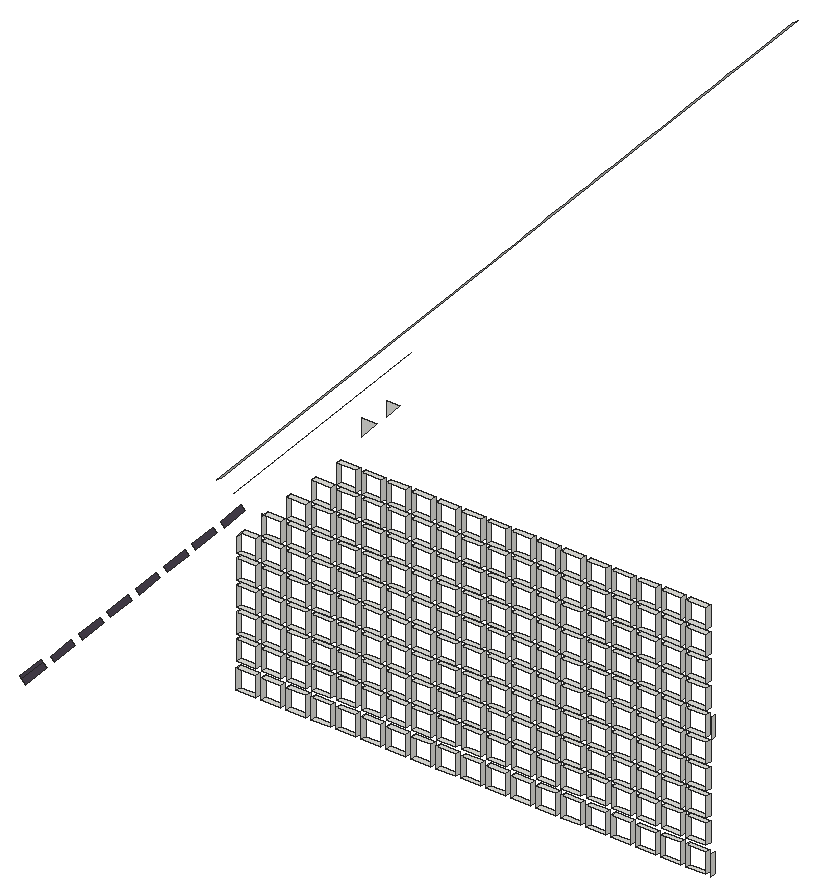
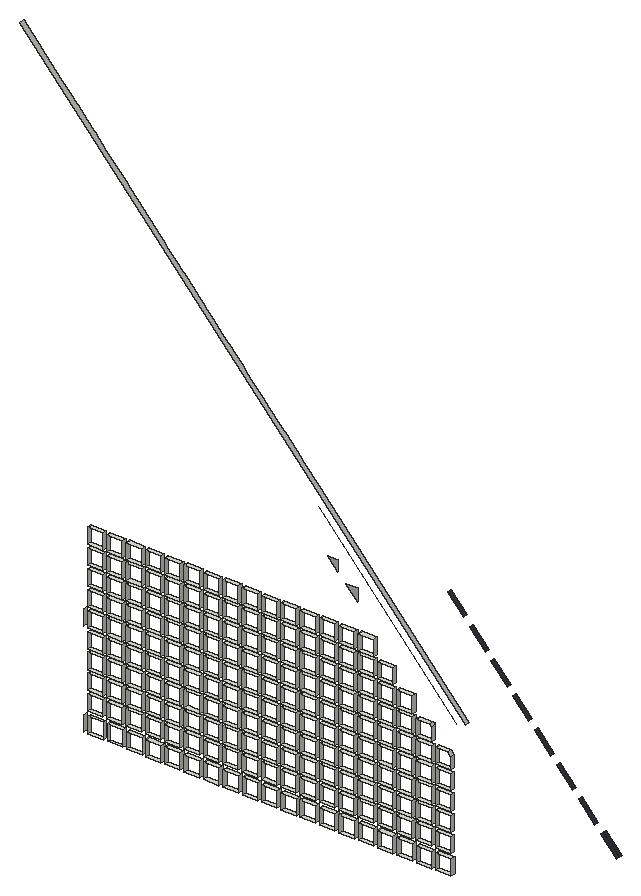
# SketchUp Ruby script. Lengths in inches.
U = 1.inch
M = Sketchup.active_model
def pt(a) = Geom::Point3d.new(a.map { |v| v * U })
def face(e, loops, mat)
  f = e.add_face(loops[0].map { |a| pt(a) })
  loops[1..].each { |l| e.add_face(l.map { |a| pt(a) }).erase! }
  f.material = f.back_material = mat if mat
  f
end
# faces: each face lists its corners as indices into pts; further lists are holes
def faces(e, pts, list, mat = nil) = list.each { |f| face(e, (f[0].is_a?(Array) ? f : [f]).map { |l| l.map { |i| pts[i] } }, mat) }
# xy, xz, yz: faces in a plane at the given z, y or x. An outline is a flat list of corners, or four numbers for a rectangle; further outlines are holes
def ring(l) = l.size == 4 ? [[l[0], l[1]], [l[2], l[1]], [l[2], l[3]], [l[0], l[3]]] : l.each_slice(2).to_a
def flat(e, list, mat, &to3) = list.each { |f| face(e, (f[0].is_a?(Array) ? f : [f]).map { |l| ring(l).map { |u, v| to3.(u, v) } }, mat) }
def xy(e, z, list, mat = nil) = flat(e, list, mat) { |x, y| [x, y, z] }
def xz(e, y, list, mat = nil) = flat(e, list, mat) { |x, z| [x, y, z] }
def yz(e, x, list, mat = nil) = flat(e, list, mat) { |y, z| [x, y, z] }
def lines(e, pts, list) = list.each { |a, b| e.add_line(pt(pts[a]), pt(pts[b])) }
# prism: a flat outline (further loops are holes) pulled along v
def prism(e, loops, v, mat = nil)
  f = face(e, loops, mat); d = Geom::Vector3d.new(v.map { |x| x * U })
  f.pushpull(f.normal.samedirection?(d) ? d.length : -d.length)
end
def box(e, o, s, mat = nil) = prism(e, [[o, [o[0] + s[0], o[1], o[2]], [o[0] + s[0], o[1] + s[1], o[2]], [o[0], o[1] + s[1], o[2]]]], [0, 0, s[2]], mat)
def at(x, y, z, deg = 0) = Geom::Transformation.translation(pt([x, y, z])) * Geom::Transformation.rotation(ORIGIN, Z_AXIS, deg.degrees)
def axes(o, x, y, z) = Geom::Transformation.new([*x, 0, *y, 0, *z, 0, *pt(o).to_a, 1])
def part(name) = M.definitions.add(name)
# library, detail: a bought-in or finely detailed component or shape, given as its bounding box
def library(name, o, s) = part(name).tap { |d| box(d.entities, o, s) }
def detail(e, o, s) = box(e.add_group.entities, o, s)
def put(e, d, t, mat = nil) = e.add_instance(d, t).tap { |i| i.material = mat if mat }
def group(e, t, mat = nil) = e.add_group.tap { |g| g.transformation = t; g.material = mat if mat }.entities
root = M.entities
M.materials.add("[Color M06]").color = [79, 71, 84]
xy(root,305.35,[[433.17,480.14,435.48,480.77],[436.08,480.14,438.39,480.77],[438.99,480.14,441.31,480.77],[441.91,480.14,444.22,480.77],[444.82,480.14,447.13,480.77],
  [447.73,480.14,450.04,480.77],[450.64,480.14,452.95,480.77],[453.55,480.14,455.87,480.77],[456.47,480.14,458.78,480.77],[459.38,480.14,461.69,480.77],
  [462.29,480.14,464.6,480.77],[465.2,480.14,467.51,480.77],[468.11,480.14,470.43,480.77],[471.03,480.14,473.34,480.77],[473.9375,480.14,476.25,480.77],
  [476.85,480.14,479.16,480.77],[479.76,480.14,482.07,480.64],[482.67,480.14,484.99,480.64],[485.59,480.14,487.9,480.64]])
xy(root,307.67,[[433.17,480.14,435.48,480.77],[436.08,480.14,438.39,480.77],[438.99,480.14,441.31,480.77],[441.91,480.14,444.22,480.77],[444.82,480.14,447.13,480.77],
  [447.73,480.14,450.04,480.77],[450.64,480.14,452.95,480.77],[453.55,480.14,455.87,480.77],[456.47,480.14,458.78,480.77],[459.38,480.14,461.69,480.77],
  [462.29,480.14,464.6,480.77],[465.2,480.14,467.51,480.77],[468.11,480.14,470.43,480.77],[471.03,480.14,473.34,480.77],[473.9375,480.14,476.25,480.77],
  [476.85,480.14,479.16,480.77],[479.76,480.14,482.07,480.64],[482.67,480.14,484.99,480.64],[485.59,480.14,487.9,480.64]])
xy(root,308.4,[[433.2,480.14,435.51,480.77],[436.11,480.14,438.42,480.77],[439.02,480.14,441.33,480.77],[441.93,480.14,444.25,480.77],[444.85,480.14,447.16,480.77],
  [447.76,480.14,450.07,480.77],[450.67,480.14,452.98,480.77],[453.58,480.14,455.89,480.77],[456.49,480.14,458.81,480.77],[459.41,480.14,461.72,480.77],
  [462.32,480.14,464.63,480.77],[465.23,480.14,467.54,480.77],[468.14,480.14,470.45,480.77],[471.05,480.14,473.37,480.77],[473.97,480.14,476.28,480.77],
  [476.88,480.14,479.19,480.77],[479.79,480.14,482.1,480.77],[482.7,480.14,485.02,480.77],[485.61,480.14,487.93,480.77]])
xy(root,310.71,[[433.2,480.14,435.51,480.77],[436.11,480.14,438.42,480.77],[439.02,480.14,441.33,480.77],[441.93,480.14,444.25,480.77],[444.85,480.14,447.16,480.77],
  [447.76,480.14,450.07,480.77],[450.67,480.14,452.98,480.77],[453.58,480.14,455.89,480.77],[456.49,480.14,458.81,480.77],[459.41,480.14,461.72,480.77],
  [462.32,480.14,464.63,480.77],[465.23,480.14,467.54,480.77],[468.14,480.14,470.45,480.77],[471.05,480.14,473.37,480.77],[473.97,480.14,476.28,480.77],
  [476.88,480.14,479.19,480.77],[479.79,480.14,482.1,480.77],[482.7,480.14,485.02,480.77],[485.61,480.14,487.93,480.77]])
xy(root,311.21,[[433.2,480.14,435.51,480.77],[436.11,480.14,438.42,480.77],[439.02,480.14,441.33,480.77],[441.93,480.14,444.25,480.77],[444.85,480.14,447.16,480.77],
  [447.76,480.14,450.07,480.77],[450.67,480.14,452.98,480.77],[453.58,480.14,455.89,480.77],[456.49,480.14,458.81,480.77],[459.41,480.14,461.72,480.77],
  [462.32,480.14,464.63,480.77],[465.23,480.14,467.54,480.77],[468.14,480.14,470.45,480.77],[471.05,480.14,473.37,480.77],[473.97,480.14,476.28,480.77],
  [476.88,480.14,479.19,480.77],[479.79,480.14,482.1,480.77],[482.7,480.14,485.02,480.77],[485.61,480.14,487.93,480.77]])
xy(root,313.52,[[433.2,480.14,435.51,480.77],[436.11,480.14,438.42,480.77],[439.02,480.14,441.33,480.77],[441.93,480.14,444.25,480.77],[444.85,480.14,447.16,480.77],
  [447.76,480.14,450.07,480.77],[450.67,480.14,452.98,480.77],[453.58,480.14,455.89,480.77],[456.49,480.14,458.81,480.77],[459.41,480.14,461.72,480.77],
  [462.32,480.14,464.63,480.77],[465.23,480.14,467.54,480.77],[468.14,480.14,470.45,480.77],[471.05,480.14,473.37,480.77],[473.97,480.14,476.28,480.77],
  [476.88,480.14,479.19,480.77],[479.79,480.14,482.1,480.77],[482.7,480.14,485.02,480.77],[485.61,480.14,487.93,480.77]])
xy(root,314.02,[[433.2,480.14,435.51,480.77],[436.11,480.14,438.42,480.77],[439.02,480.14,441.33,480.77],[441.93,480.14,444.25,480.77],[444.85,480.14,447.16,480.77],
  [447.76,480.14,450.07,480.77],[450.67,480.14,452.98,480.77],[453.58,480.14,455.89,480.77],[456.49,480.14,458.81,480.77],[459.41,480.14,461.72,480.77],
  [462.32,480.14,464.63,480.77],[465.23,480.14,467.54,480.77],[468.14,480.14,470.45,480.77],[471.05,480.14,473.37,480.77],[473.97,480.14,476.28,480.77],
  [476.88,480.14,479.19,480.77],[479.79,480.14,482.1,480.77],[482.7,480.14,485.02,480.77],[485.61,480.14,487.93,480.77]])
xy(root,316.34,[[433.2,480.14,435.51,480.77],[436.11,480.14,438.42,480.77],[439.02,480.14,441.33,480.77],[441.93,480.14,444.25,480.77],[444.85,480.14,447.16,480.77],
  [447.76,480.14,450.07,480.77],[450.67,480.14,452.98,480.77],[453.58,480.14,455.89,480.77],[456.49,480.14,458.81,480.77],[459.41,480.14,461.72,480.77],
  [462.32,480.14,464.63,480.77],[465.23,480.14,467.54,480.77],[468.14,480.14,470.45,480.77],[471.05,480.14,473.37,480.77],[473.97,480.14,476.28,480.77],
  [476.88,480.14,479.19,480.77],[479.79,480.14,482.1,480.77],[482.7,480.14,485.02,480.77],[485.61,480.14,487.93,480.77]])
xy(root,316.84,[[433.2,480.14,435.51,480.77],[436.11,480.14,438.42,480.77],[439.02,480.14,441.33,480.77],[441.93,480.14,444.25,480.77],[444.85,480.14,447.16,480.77],
  [447.76,480.14,450.07,480.77],[450.67,480.14,452.98,480.77],[453.58,480.14,455.89,480.77],[456.49,480.14,458.81,480.77],[459.41,480.14,461.72,480.77],
  [462.32,480.14,464.63,480.77],[465.23,480.14,467.54,480.77],[468.14,480.14,470.45,480.77],[471.05,480.14,473.37,480.77],[473.97,480.14,476.28,480.77],
  [476.88,480.14,479.19,480.77],[479.79,480.14,482.1,480.77],[482.7,480.14,485.02,480.77],[485.61,480.14,487.93,480.77]])
xy(root,319.15,[[433.2,480.14,435.51,480.77],[436.11,480.14,438.42,480.77],[439.02,480.14,441.33,480.77],[441.93,480.14,444.25,480.77],[444.85,480.14,447.16,480.77],
  [447.76,480.14,450.07,480.77],[450.67,480.14,452.98,480.77],[453.58,480.14,455.89,480.77],[456.49,480.14,458.81,480.77],[459.41,480.14,461.72,480.77],
  [462.32,480.14,464.63,480.77],[465.23,480.14,467.54,480.77],[468.14,480.14,470.45,480.77],[471.05,480.14,473.37,480.77],[473.97,480.14,476.28,480.77],
  [476.88,480.14,479.19,480.77],[479.79,480.14,482.1,480.77],[482.7,480.14,485.02,480.77],[485.61,480.14,487.93,480.77]])
xy(root,319.65,[[433.2,480.14,435.51,480.77],[436.11,480.14,438.42,480.77],[439.02,480.14,441.33,480.77],[441.93,480.14,444.25,480.77],[444.85,480.14,447.16,480.77],
  [447.76,480.14,450.07,480.77],[450.67,480.14,452.98,480.77],[453.58,480.14,455.89,480.77],[456.49,480.14,458.81,480.77],[459.41,480.14,461.72,480.77],
  [462.32,480.14,464.63,480.77],[465.23,480.14,467.54,480.77],[468.14,480.14,470.45,480.77],[471.05,480.14,473.37,480.77],[473.97,480.14,476.28,480.77],
  [476.88,480.14,479.19,480.77],[479.79,480.14,482.1,480.77],[482.7,480.14,485.02,480.77],[485.61,480.14,487.93,480.7]])
xy(root,321.96,[[433.73,480.14,435.51,480.77],[436.11,480.14,438.42,480.77],[439.02,480.14,441.33,480.77],[441.93,480.14,444.25,480.77],[444.85,480.14,447.16,480.77],
  [447.76,480.14,450.07,480.77],[450.67,480.14,452.98,480.77],[453.58,480.14,455.89,480.77],[456.49,480.14,458.81,480.77],[459.41,480.14,461.72,480.77],
  [462.32,480.14,464.63,480.77],[465.23,480.14,467.54,480.77],[468.14,480.14,470.45,480.77],[471.05,480.14,473.37,480.77],[473.97,480.14,476.28,480.77],
  [476.88,480.14,479.19,480.77],[479.79,480.14,482.1,480.77],[482.7,480.14,485.02,480.77],[485.61,480.14,487.93,480.7]])
xy(root,322.46,[[436.11,480.14,438.42,480.77],[439.02,480.14,441.33,480.77],[441.93,480.14,444.25,480.77],[444.85,480.14,447.16,480.77],[447.76,480.14,450.07,480.77],
  [450.67,480.14,452.98,480.77],[453.58,480.14,455.89,480.77],[456.49,480.14,458.81,480.77],[459.41,480.14,461.72,480.77],[462.32,480.14,464.63,480.77],
  [465.23,480.14,467.54,480.77],[468.14,480.14,470.45,480.77],[471.05,480.14,473.37,480.77],[473.97,480.14,476.28,480.77],[476.88,480.14,479.19,480.77],
  [479.79,480.14,482.1,480.77],[482.7,480.14,485.02,480.77],[485.61,480.14,487.93,480.77]])
xy(root,324.77,[[436.37,480.14,438.42,480.77],[439.02,480.14,441.33,480.77],[441.93,480.14,444.25,480.77],[444.85,480.14,447.16,480.77],[447.76,480.14,450.07,480.77],
  [450.67,480.14,452.98,480.77],[453.58,480.14,455.89,480.77],[456.49,480.14,458.81,480.77],[459.41,480.14,461.72,480.77],[462.32,480.14,464.63,480.77],
  [465.23,480.14,467.54,480.77],[468.14,480.14,470.45,480.77],[471.05,480.14,473.37,480.77],[473.97,480.14,476.28,480.77],[476.88,480.14,479.19,480.77],
  [479.79,480.14,482.1,480.77],[482.7,480.14,485.02,480.77],[485.61,480.14,487.93,480.77]])
xy(root,325.27,[[439.02,480.14,441.33,480.77],[441.93,480.14,444.25,480.77],[444.85,480.14,447.16,480.77],[447.76,480.14,450.07,480.77],[450.67,480.14,452.98,480.77],
  [453.58,480.14,455.89,480.77],[456.49,480.14,458.81,480.77],[459.41,480.14,461.72,480.77],[462.32,480.14,464.63,480.77],[465.23,480.14,467.54,480.77],
  [468.14,480.14,470.45,480.77],[471.05,480.14,473.37,480.77],[473.97,480.14,476.28,480.77],[476.88,480.14,479.19,480.77],[479.79,480.14,482.1,480.77],
  [482.7,480.14,485.02,480.77],[485.61,480.14,487.93,480.77]])
xy(root,327.59,[[439.02,480.14,441.33,480.77],[441.93,480.14,444.25,480.77],[444.85,480.14,447.16,480.77],[447.76,480.14,450.07,480.77],[450.67,480.14,452.98,480.77],
  [453.58,480.14,455.89,480.77],[456.49,480.14,458.81,480.77],[459.41,480.14,461.72,480.77],[462.32,480.14,464.63,480.77],[465.23,480.14,467.54,480.77],
  [468.14,480.14,470.45,480.77],[471.05,480.14,473.37,480.77],[473.97,480.14,476.28,480.77],[476.88,480.14,479.19,480.77],[479.79,480.14,482.1,480.77],
  [482.7,480.14,485.02,480.77],[485.61,480.14,487.93,480.77]])
xy(root,328.09,[[441.93,480.14,444.25,480.77],[444.85,480.14,447.16,480.77],[447.76,480.14,450.07,480.77],[450.67,480.14,452.98,480.77],[453.58,480.14,455.89,480.77],
  [456.49,480.14,458.81,480.77],[459.41,480.14,461.72,480.77],[462.32,480.14,464.63,480.77],[465.23,480.14,467.54,480.77],[468.14,480.14,470.45,480.77],
  [471.05,480.14,473.37,480.77],[473.97,480.14,476.28,480.77],[476.88,480.14,479.19,480.77],[479.79,480.14,482.1,480.77],[482.7,480.14,485.02,480.77],
  [485.61,480.14,487.93,480.77]])
xy(root,330.4,[[441.93,480.14,444.25,480.77],[444.85,480.14,447.16,480.77],[447.76,480.14,450.07,480.77],[450.67,480.14,452.98,480.77],[453.58,480.14,455.89,480.77],
  [456.49,480.14,458.81,480.77],[459.41,480.14,461.72,480.77],[462.32,480.14,464.63,480.77],[465.23,480.14,467.54,480.77],[468.14,480.14,470.45,480.77],
  [471.05,480.14,473.37,480.77],[473.97,480.14,476.28,480.77],[476.88,480.14,479.19,480.77],[479.79,480.14,482.1,480.77],[482.7,480.14,485.02,480.77],
  [485.61,480.14,487.93,480.77]])
xy(root,330.9,[[444.85,480.14,447.16,480.77],[447.76,480.14,450.07,480.77],[450.67,480.14,452.98,480.77],[453.58,480.14,455.89,480.77],[456.49,480.14,458.81,480.77],
  [459.41,480.14,461.72,480.77],[462.32,480.14,464.63,480.77],[465.23,480.14,467.54,480.77],[468.14,480.14,470.45,480.77],[471.05,480.14,473.37,480.77],
  [473.97,480.14,476.28,480.77],[476.88,480.14,479.19,480.77],[479.79,480.14,482.1,480.77],[482.7,480.14,485.02,480.77],[485.61,480.14,487.93,480.77]])
xy(root,333.21,[[444.85,480.14,447.16,480.77],[447.76,480.14,450.07,480.77],[450.67,480.14,452.98,480.77],[453.58,480.14,455.89,480.77],[456.49,480.14,458.81,480.77],
  [459.41,480.14,461.72,480.77],[462.32,480.14,464.63,480.77],[465.23,480.14,467.54,480.77],[468.14,480.14,470.45,480.77],[471.05,480.14,473.37,480.77],
  [473.97,480.14,476.28,480.77],[476.88,480.14,479.19,480.77],[479.79,480.14,482.1,480.77],[482.7,480.14,485.02,480.77],[485.61,480.14,487.93,480.77]])
xz(root,467.1875,[[419.07,306.65,421.49,309.22,421.04,309.65,418.61,307.08],[418.61,307.08,421.04,309.65,420.81,309.87,418.39,307.29],[422.37,310.16,424.79,312.73,424.33,313.16,421.91,310.59],[425.67,313.66,428.09,316.23,427.63,316.66,425.21,314.09],[428.96,317.17,431.39,319.74,430.93,320.17,428.51,317.59],
  [432.26,320.67,434.68,323.24,434.23,323.67,431.81,321.1],[435.5625,324.17,437.98,326.75,437.53,327.17,435.11,324.6],[438.86,327.68,441.28,330.25,440.83,330.68,438.41,328.11],[442.16,331.18,444.58,333.75,444.125,334.18,441.7,331.61]],"[Color M06]")
xz(root,480.14,[[436.11,324.5,436.37,324.77,436.11,324.77],[447.76,336.93,449.55,338.84,447.76,338.84],[450.67,340.04,452.18,341.65,450.67,341.65]])
yz(root,433.17,[[480.14,305.35,480.77,307.67]])
yz(root,433.2,[[480.14,308.4,480.77,310.71],[480.14,311.21,480.77,313.52],[480.14,314.02,480.77,316.34],[480.14,316.84,480.77,319.15],[480.14,319.65,480.77,321.39]])
yz(root,435.48,[[480.14,305.35,480.77,307.67]])
yz(root,435.51,[[480.14,308.4,480.77,310.71],[480.14,311.21,480.77,313.52],[480.14,314.02,480.77,316.34],[480.14,316.84,480.77,319.15],[480.14,319.65,480.77,321.96]])
yz(root,436.08,[[480.14,305.35,480.77,307.67]])
yz(root,436.11,[[480.14,308.4,480.77,310.71],[480.14,311.21,480.77,313.52],[480.14,314.02,480.77,316.34],[480.14,316.84,480.77,319.15],[480.14,319.65,480.77,321.96],
  [480.14,322.46,480.77,324.5]])
yz(root,438.39,[[480.14,305.35,480.77,307.67]])
yz(root,438.42,[[480.14,308.4,480.77,310.71],[480.14,311.21,480.77,313.52],[480.14,314.02,480.77,316.34],[480.14,316.84,480.77,319.15],[480.14,319.65,480.77,321.96],
  [480.14,322.46,480.77,324.77]])
yz(root,438.99,[[480.14,305.35,480.77,307.67]])
yz(root,439.02,[[480.14,308.4,480.77,310.71],[480.14,311.21,480.77,313.52],[480.14,314.02,480.77,316.34],[480.14,316.84,480.77,319.15],[480.14,319.65,480.77,321.96],
  [480.14,322.46,480.77,324.77],[480.14,325.27,480.77,327.59]])
yz(root,441.31,[[480.14,305.35,480.77,307.67]])
yz(root,441.33,[[480.14,308.4,480.77,310.71],[480.14,311.21,480.77,313.52],[480.14,314.02,480.77,316.34],[480.14,316.84,480.77,319.15],[480.14,319.65,480.77,321.96],
  [480.14,322.46,480.77,324.77],[480.14,325.27,480.77,327.59]])
yz(root,441.91,[[480.14,305.35,480.77,307.67]])
yz(root,441.93,[[480.14,308.4,480.77,310.71],[480.14,311.21,480.77,313.52],[480.14,314.02,480.77,316.34],[480.14,316.84,480.77,319.15],[480.14,319.65,480.77,321.96],
  [480.14,322.46,480.77,324.77],[480.14,325.27,480.77,327.59],[480.14,328.09,480.77,330.4]])
yz(root,444.22,[[480.14,305.35,480.77,307.67]])
yz(root,444.25,[[480.14,308.4,480.77,310.71],[480.14,311.21,480.77,313.52],[480.14,314.02,480.77,316.34],[480.14,316.84,480.77,319.15],[480.14,319.65,480.77,321.96],
  [480.14,322.46,480.77,324.77],[480.14,325.27,480.77,327.59],[480.14,328.09,480.77,330.4]])
yz(root,444.82,[[480.14,305.35,480.77,307.67]])
yz(root,444.85,[[480.14,308.4,480.77,310.71],[480.14,311.21,480.77,313.52],[480.14,314.02,480.77,316.34],[480.14,316.84,480.77,319.15],[480.14,319.65,480.77,321.96],
  [480.14,322.46,480.77,324.77],[480.14,325.27,480.77,327.59],[480.14,328.09,480.77,330.4],[480.14,330.9,480.77,333.21]])
yz(root,447.13,[[480.14,305.35,480.77,307.67]])
yz(root,447.16,[[480.14,308.4,480.77,310.71],[480.14,311.21,480.77,313.52],[480.14,314.02,480.77,316.34],[480.14,316.84,480.77,319.15],[480.14,319.65,480.77,321.96],
  [480.14,322.46,480.77,324.77],[480.14,325.27,480.77,327.59],[480.14,328.09,480.77,330.4],[480.14,330.9,480.77,333.21]])
yz(root,447.73,[[480.14,305.35,480.77,307.67]])
yz(root,447.76,[[480.14,308.4,480.77,310.71],[480.14,311.21,480.77,313.52],[480.14,314.02,480.77,316.34],[480.14,316.84,480.77,319.15],[480.14,319.65,480.77,321.96],
  [480.14,322.46,480.77,324.77],[480.14,325.27,480.77,327.59],[480.14,328.09,480.77,330.4],[480.14,330.9,480.77,333.21]])
yz(root,450.04,[[480.14,305.35,480.77,307.67]])
yz(root,450.07,[[480.14,308.4,480.77,310.71],[480.14,311.21,480.77,313.52],[480.14,314.02,480.77,316.34],[480.14,316.84,480.77,319.15],[480.14,319.65,480.77,321.96],
  [480.14,322.46,480.77,324.77],[480.14,325.27,480.77,327.59],[480.14,328.09,480.77,330.4],[480.14,330.9,480.77,333.21]])
yz(root,450.64,[[480.14,305.35,480.77,307.67]])
yz(root,450.67,[[480.14,308.4,480.77,310.71],[480.14,311.21,480.77,313.52],[480.14,314.02,480.77,316.34],[480.14,316.84,480.77,319.15],[480.14,319.65,480.77,321.96],
  [480.14,322.46,480.77,324.77],[480.14,325.27,480.77,327.59],[480.14,328.09,480.77,330.4],[480.14,330.9,480.77,333.21]])
yz(root,452.95,[[480.14,305.35,480.77,307.67]])
yz(root,452.98,[[480.14,308.4,480.77,310.71],[480.14,311.21,480.77,313.52],[480.14,314.02,480.77,316.34],[480.14,316.84,480.77,319.15],[480.14,319.65,480.77,321.96],
  [480.14,322.46,480.77,324.77],[480.14,325.27,480.77,327.59],[480.14,328.09,480.77,330.4],[480.14,330.9,480.77,333.21]])
yz(root,453.55,[[480.14,305.35,480.77,307.67]])
yz(root,453.58,[[480.14,308.4,480.77,310.71],[480.14,311.21,480.77,313.52],[480.14,314.02,480.77,316.34],[480.14,316.84,480.77,319.15],[480.14,319.65,480.77,321.96],
  [480.14,322.46,480.77,324.77],[480.14,325.27,480.77,327.59],[480.14,328.09,480.77,330.4],[480.14,330.9,480.77,333.21]])
yz(root,455.87,[[480.14,305.35,480.77,307.67]])
yz(root,455.89,[[480.14,308.4,480.77,310.71],[480.14,311.21,480.77,313.52],[480.14,314.02,480.77,316.34],[480.14,316.84,480.77,319.15],[480.14,319.65,480.77,321.96],
  [480.14,322.46,480.77,324.77],[480.14,325.27,480.77,327.59],[480.14,328.09,480.77,330.4],[480.14,330.9,480.77,333.21]])
yz(root,456.47,[[480.14,305.35,480.77,307.67]])
yz(root,456.49,[[480.14,308.4,480.77,310.71],[480.14,311.21,480.77,313.52],[480.14,314.02,480.77,316.34],[480.14,316.84,480.77,319.15],[480.14,319.65,480.77,321.96],
  [480.14,322.46,480.77,324.77],[480.14,325.27,480.77,327.59],[480.14,328.09,480.77,330.4],[480.14,330.9,480.77,333.21]])
yz(root,458.78,[[480.14,305.35,480.77,307.67]])
yz(root,458.81,[[480.14,308.4,480.77,310.71],[480.14,311.21,480.77,313.52],[480.14,314.02,480.77,316.34],[480.14,316.84,480.77,319.15],[480.14,319.65,480.77,321.96],
  [480.14,322.46,480.77,324.77],[480.14,325.27,480.77,327.59],[480.14,328.09,480.77,330.4],[480.14,330.9,480.77,333.21]])
yz(root,459.38,[[480.14,305.35,480.77,307.67]])
yz(root,459.41,[[480.14,308.4,480.77,310.71],[480.14,311.21,480.77,313.52],[480.14,314.02,480.77,316.34],[480.14,316.84,480.77,319.15],[480.14,319.65,480.77,321.96],
  [480.14,322.46,480.77,324.77],[480.14,325.27,480.77,327.59],[480.14,328.09,480.77,330.4],[480.14,330.9,480.77,333.21]])
yz(root,461.69,[[480.14,305.35,480.77,307.67]])
yz(root,461.72,[[480.14,308.4,480.77,310.71],[480.14,311.21,480.77,313.52],[480.14,314.02,480.77,316.34],[480.14,316.84,480.77,319.15],[480.14,319.65,480.77,321.96],
  [480.14,322.46,480.77,324.77],[480.14,325.27,480.77,327.59],[480.14,328.09,480.77,330.4],[480.14,330.9,480.77,333.21]])
yz(root,462.29,[[480.14,305.35,480.77,307.67]])
yz(root,462.32,[[480.14,308.4,480.77,310.71],[480.14,311.21,480.77,313.52],[480.14,314.02,480.77,316.34],[480.14,316.84,480.77,319.15],[480.14,319.65,480.77,321.96],
  [480.14,322.46,480.77,324.77],[480.14,325.27,480.77,327.59],[480.14,328.09,480.77,330.4],[480.14,330.9,480.77,333.21]])
yz(root,464.6,[[480.14,305.35,480.77,307.67]])
yz(root,464.63,[[480.14,308.4,480.77,310.71],[480.14,311.21,480.77,313.52],[480.14,314.02,480.77,316.34],[480.14,316.84,480.77,319.15],[480.14,319.65,480.77,321.96],
  [480.14,322.46,480.77,324.77],[480.14,325.27,480.77,327.59],[480.14,328.09,480.77,330.4],[480.14,330.9,480.77,333.21]])
yz(root,465.2,[[480.14,305.35,480.77,307.67]])
yz(root,465.23,[[480.14,308.4,480.77,310.71],[480.14,311.21,480.77,313.52],[480.14,314.02,480.77,316.34],[480.14,316.84,480.77,319.15],[480.14,319.65,480.77,321.96],
  [480.14,322.46,480.77,324.77],[480.14,325.27,480.77,327.59],[480.14,328.09,480.77,330.4],[480.14,330.9,480.77,333.21]])
yz(root,467.51,[[480.14,305.35,480.77,307.67]])
yz(root,467.54,[[480.14,308.4,480.77,310.71],[480.14,311.21,480.77,313.52],[480.14,314.02,480.77,316.34],[480.14,316.84,480.77,319.15],[480.14,319.65,480.77,321.96],
  [480.14,322.46,480.77,324.77],[480.14,325.27,480.77,327.59],[480.14,328.09,480.77,330.4],[480.14,330.9,480.77,333.21]])
yz(root,468.11,[[480.14,305.35,480.77,307.67]])
yz(root,468.14,[[480.14,308.4,480.77,310.71],[480.14,311.21,480.77,313.52],[480.14,314.02,480.77,316.34],[480.14,316.84,480.77,319.15],[480.14,319.65,480.77,321.96],
  [480.14,322.46,480.77,324.77],[480.14,325.27,480.77,327.59],[480.14,328.09,480.77,330.4],[480.14,330.9,480.77,333.21]])
yz(root,470.43,[[480.14,305.35,480.77,307.67]])
yz(root,470.45,[[480.14,308.4,480.77,310.71],[480.14,311.21,480.77,313.52],[480.14,314.02,480.77,316.34],[480.14,316.84,480.77,319.15],[480.14,319.65,480.77,321.96],
  [480.14,322.46,480.77,324.77],[480.14,325.27,480.77,327.59],[480.14,328.09,480.77,330.4],[480.14,330.9,480.77,333.21]])
yz(root,471.03,[[480.14,305.35,480.77,307.67]])
yz(root,471.05,[[480.14,308.4,480.77,310.71],[480.14,311.21,480.77,313.52],[480.14,314.02,480.77,316.34],[480.14,316.84,480.77,319.15],[480.14,319.65,480.77,321.96],
  [480.14,322.46,480.77,324.77],[480.14,325.27,480.77,327.59],[480.14,328.09,480.77,330.4],[480.14,330.9,480.77,333.21]])
yz(root,473.34,[[480.14,305.35,480.77,307.67]])
yz(root,473.37,[[480.14,308.4,480.77,310.71],[480.14,311.21,480.77,313.52],[480.14,314.02,480.77,316.34],[480.14,316.84,480.77,319.15],[480.14,319.65,480.77,321.96],
  [480.14,322.46,480.77,324.77],[480.14,325.27,480.77,327.59],[480.14,328.09,480.77,330.4],[480.14,330.9,480.77,333.21]])
yz(root,473.9375,[[480.14,305.35,480.77,307.67]])
yz(root,473.97,[[480.14,308.4,480.77,310.71],[480.14,311.21,480.77,313.52],[480.14,314.02,480.77,316.34],[480.14,316.84,480.77,319.15],[480.14,319.65,480.77,321.96],
  [480.14,322.46,480.77,324.77],[480.14,325.27,480.77,327.59],[480.14,328.09,480.77,330.4],[480.14,330.9,480.77,333.21]])
yz(root,476.25,[[480.14,305.35,480.77,307.67]])
yz(root,476.28,[[480.14,308.4,480.77,310.71],[480.14,311.21,480.77,313.52],[480.14,314.02,480.77,316.34],[480.14,316.84,480.77,319.15],[480.14,319.65,480.77,321.96],
  [480.14,322.46,480.77,324.77],[480.14,325.27,480.77,327.59],[480.14,328.09,480.77,330.4],[480.14,330.9,480.77,333.21]])
yz(root,476.85,[[480.14,305.35,480.77,307.67]])
yz(root,476.88,[[480.14,308.4,480.77,310.71],[480.14,311.21,480.77,313.52],[480.14,314.02,480.77,316.34],[480.14,316.84,480.77,319.15],[480.14,319.65,480.77,321.96],
  [480.14,322.46,480.77,324.77],[480.14,325.27,480.77,327.59],[480.14,328.09,480.77,330.4],[480.14,330.9,480.77,333.21]])
yz(root,479.16,[[480.14,305.35,480.77,307.67]])
yz(root,479.19,[[480.14,308.4,480.77,310.71],[480.14,311.21,480.77,313.52],[480.14,314.02,480.77,316.34],[480.14,316.84,480.77,319.15],[480.14,319.65,480.77,321.96],
  [480.14,322.46,480.77,324.77],[480.14,325.27,480.77,327.59],[480.14,328.09,480.77,330.4],[480.14,330.9,480.77,333.21]])
yz(root,479.76,[[480.14,305.35,480.64,307.67]])
yz(root,479.79,[[480.14,308.4,480.77,310.71],[480.14,311.21,480.77,313.52],[480.14,314.02,480.77,316.34],[480.14,316.84,480.77,319.15],[480.14,319.65,480.77,321.96],
  [480.14,322.46,480.77,324.77],[480.14,325.27,480.77,327.59],[480.14,328.09,480.77,330.4],[480.14,330.9,480.77,333.21]])
yz(root,482.07,[[480.14,305.35,480.64,307.67]])
yz(root,482.1,[[480.14,308.4,480.77,310.71],[480.14,311.21,480.77,313.52],[480.14,314.02,480.77,316.34],[480.14,316.84,480.77,319.15],[480.14,319.65,480.77,321.96],
  [480.14,322.46,480.77,324.77],[480.14,325.27,480.77,327.59],[480.14,328.09,480.77,330.4],[480.14,330.9,480.77,333.21]])
yz(root,482.67,[[480.14,305.35,480.64,307.67]])
yz(root,482.7,[[480.14,308.4,480.77,310.71],[480.14,311.21,480.77,313.52],[480.14,314.02,480.77,316.34],[480.14,316.84,480.77,319.15],[480.14,319.65,480.77,321.96],
  [480.14,322.46,480.77,324.77],[480.14,325.27,480.77,327.59],[480.14,328.09,480.77,330.4],[480.14,330.9,480.77,333.21]])
yz(root,484.99,[[480.14,305.35,480.64,307.67]])
yz(root,485.02,[[480.14,308.4,480.77,310.71],[480.14,311.21,480.77,313.52],[480.14,314.02,480.77,316.34],[480.14,316.84,480.77,319.15],[480.14,319.65,480.77,321.96],
  [480.14,322.46,480.77,324.77],[480.14,325.27,480.77,327.59],[480.14,328.09,480.77,330.4],[480.14,330.9,480.77,333.21]])
yz(root,485.59,[[480.14,305.35,480.64,307.67]])
yz(root,485.61,[[480.14,308.4,480.77,310.71],[480.14,311.21,480.77,313.52],[480.14,314.02,480.77,316.34],[480.14,316.84,480.77,319.15],[480.14,319.65,480.7,321.96],
  [480.14,322.46,480.77,324.77],[480.14,325.27,480.77,327.59],[480.14,328.09,480.77,330.4],[480.14,330.9,480.77,333.21]])
yz(root,487.9,[[480.14,305.35,480.64,307.67]])
yz(root,487.93,[[480.14,308.4,480.77,310.71],[480.14,311.21,480.77,313.52],[480.14,314.02,480.77,316.34],[480.14,316.84,480.77,319.15],[480.14,319.65,480.7,321.96],
  [480.14,322.46,480.77,324.77],[480.14,325.27,480.77,327.59],[480.14,328.09,480.77,330.4],[480.14,330.9,480.77,333.21]])
yz(root,488.5,[[480.14,305.35,480.64,307.67]])
yz(root,488.53,[[480.14,319.65,480.7,321.96]])
p = [[433.73,480.14,321.96],[433.2,480.14,321.39],[433.2,480.77,321.39],[433.73,480.77,321.96],[436.37,480.14,324.77],[436.11,480.14,324.5],
  [436.11,480.77,324.5],[436.37,480.77,324.77],[492.53,480.14,391.9],[498.04,480.14,397.75],[498.04,480.77,397.75],[430.97,480.77,326.5],
  [430.97,480.14,326.5],[453.64,480.14,350.59],[455.82,480.14,352.9],[456.49,480.14,353.62],[458.47,480.14,355.71],[459.41,480.14,356.71],
  [461.11,480.14,358.52],[461.59,480.14,359.02],[461.72,480.14,359.17],[462.32,480.14,359.8],[463.76,480.14,361.34],[464.23,480.14,361.84],
  [464.63,480.14,362.26],[465.23,480.14,362.9],[466.41,480.14,364.15],[466.88,480.14,364.65],[467.54,480.14,365.35],[468.14,480.14,365.99],
  [469.06,480.14,366.96],[469.53,480.14,367.46],[470.45,480.14,368.45],[471.05,480.14,369.08],[471.7,480.14,369.77],[472.18,480.14,370.27],
  [473.37,480.14,371.54],[473.97,480.14,372.18],[474.35,480.14,372.59],[474.82,480.14,373.09],[476.28,480.14,374.63],[476.88,480.14,375.27],
  [477,480.14,375.4],[477.41,480.14,375.84],[479.19,480.14,377.73],[480,480.14,378.59],[482.1,480.14,380.82],[482.7,480.14,381.46],
  [484.77,480.14,383.65],[485.61,480.14,384.55],[487.35,480.14,386.4],[487.77,480.14,386.84],[487.93,480.14,387.01],[488.53,480.14,387.65],
  [489.94,480.14,389.15],[490.35,480.14,389.59],[490.84,480.14,390.1],[491.4375,480.14,390.74],[453.59,480.14,347.77],[432.86,480.14,325.75]]
faces(root,p,[[0,1,2,3],[4,5,6,7],[8,9,10,11,12,13,14,15,16,17,18,19,20,21,22,23,24,25,26,27,28,29,30,31,32,33,34,35,36,37,38,39,40,41,42,43,44,45,46,47,48,49,50,51,52,53,54,55,56,57]])
lines(root,p,[[58,59]])
